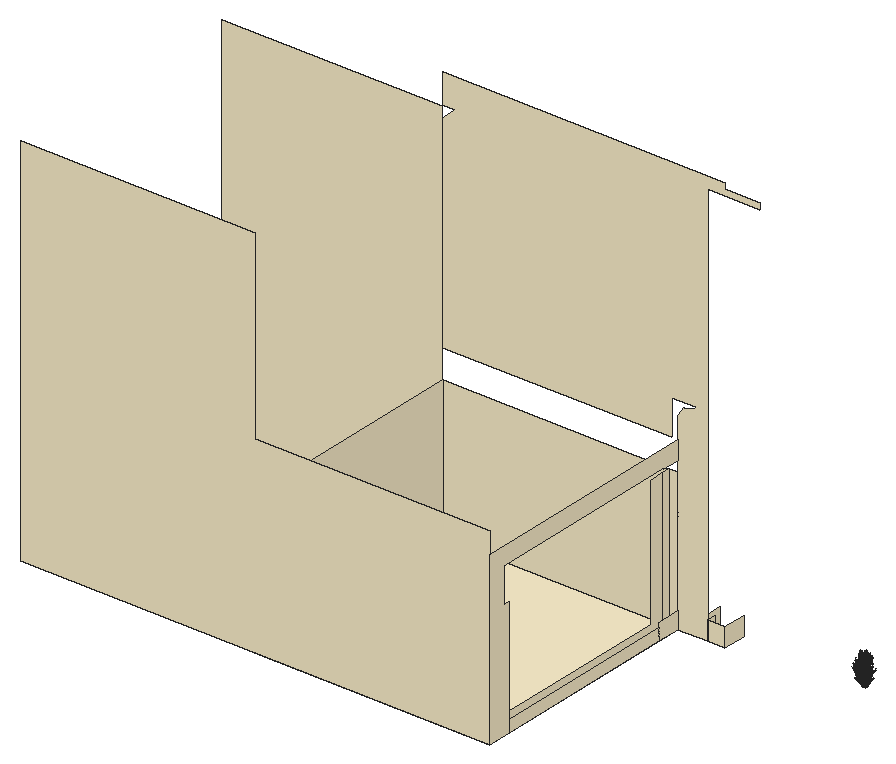
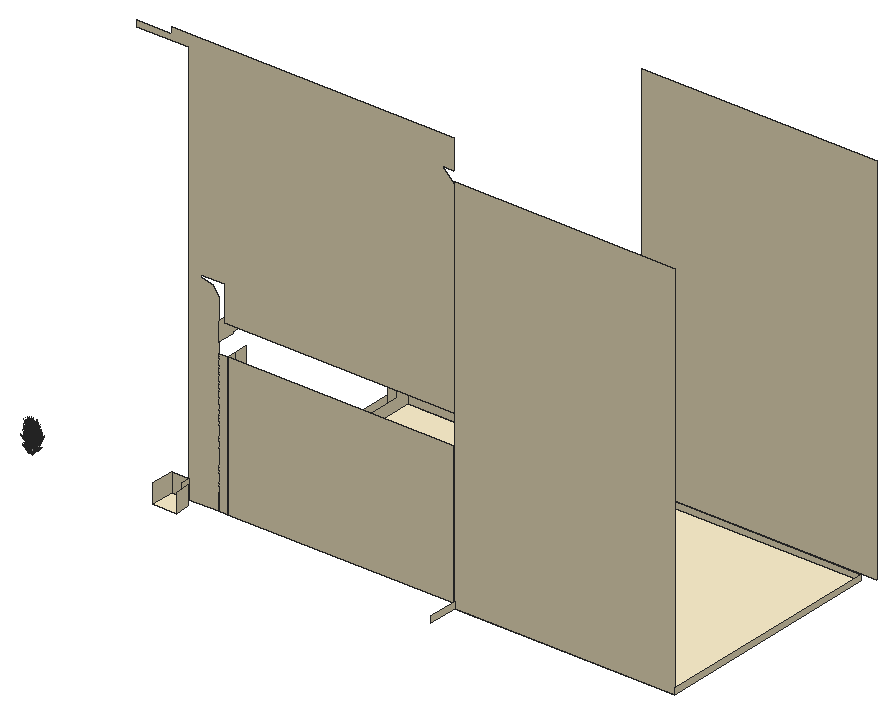
# SketchUp Ruby script. Lengths in inches.
U = 1.inch
M = Sketchup.active_model
def pt(a) = Geom::Point3d.new(a.map { |v| v * U })
def face(e, loops, mat)
  f = e.add_face(loops[0].map { |a| pt(a) })
  loops[1..].each { |l| e.add_face(l.map { |a| pt(a) }).erase! }
  f.material = f.back_material = mat if mat
  f
end
# faces: each face lists its corners as indices into pts; further lists are holes
def faces(e, pts, list, mat = nil) = list.each { |f| face(e, (f[0].is_a?(Array) ? f : [f]).map { |l| l.map { |i| pts[i] } }, mat) }
# xy, xz, yz: faces in a plane at the given z, y or x. An outline is a flat list of corners, or four numbers for a rectangle; further outlines are holes
def ring(l) = l.size == 4 ? [[l[0], l[1]], [l[2], l[1]], [l[2], l[3]], [l[0], l[3]]] : l.each_slice(2).to_a
def flat(e, list, mat, &to3) = list.each { |f| face(e, (f[0].is_a?(Array) ? f : [f]).map { |l| ring(l).map { |u, v| to3.(u, v) } }, mat) }
def xy(e, z, list, mat = nil) = flat(e, list, mat) { |x, y| [x, y, z] }
def xz(e, y, list, mat = nil) = flat(e, list, mat) { |x, z| [x, y, z] }
def yz(e, x, list, mat = nil) = flat(e, list, mat) { |y, z| [x, y, z] }
def lines(e, pts, list) = list.each { |a, b| e.add_line(pt(pts[a]), pt(pts[b])) }
# prism: a flat outline (further loops are holes) pulled along v
def prism(e, loops, v, mat = nil)
  f = face(e, loops, mat); d = Geom::Vector3d.new(v.map { |x| x * U })
  f.pushpull(f.normal.samedirection?(d) ? d.length : -d.length)
end
def box(e, o, s, mat = nil) = prism(e, [[o, [o[0] + s[0], o[1], o[2]], [o[0] + s[0], o[1] + s[1], o[2]], [o[0], o[1] + s[1], o[2]]]], [0, 0, s[2]], mat)
def at(x, y, z, deg = 0) = Geom::Transformation.translation(pt([x, y, z])) * Geom::Transformation.rotation(ORIGIN, Z_AXIS, deg.degrees)
def axes(o, x, y, z) = Geom::Transformation.new([*x, 0, *y, 0, *z, 0, *pt(o).to_a, 1])
def part(name) = M.definitions.add(name)
# library, detail: a bought-in or finely detailed component or shape, given as its bounding box
def library(name, o, s) = part(name).tap { |d| box(d.entities, o, s) }
def detail(e, o, s) = box(e.add_group.entities, o, s)
def put(e, d, t, mat = nil) = e.add_instance(d, t).tap { |i| i.material = mat if mat }
def group(e, t, mat = nil) = e.add_group.tap { |g| g.transformation = t; g.material = mat if mat }.entities
root = M.entities
M.materials.add("D01_Frost_White").color = [255, 242, 206]
M.materials.add("LightPink_Translucent").color = [144, 107, 117]
M.materials["LightPink_Translucent"].alpha = 0.75
c1 = part("blade")
p = [[2.15,0.21,22],[0,0.17,0],[0.09,0.45,0],[2.18,0.31,22],[2.29,0.31,22],[0.38,0.45,0],
  [2.48,0.24,33],[2.49,0.24,33],[2.48,0.22,33]]
faces(c1.entities,p,[[0,1,2,3],[4,5,2,3],[6,3,4,7],[8,0,3,6]])
c2 = part("seeds")
p = [[0.3,-0.1,1.38],[-0.01,-0.03,1.59],[-0.01,-0.03,0.03],[0.14,-0.07,-0.07],[0.29,-0.03,3],[0.15,0.01,3.11]]
faces(c2.entities,p,[[0,1,2,3],[1,0,4,5]],"LightPink_Translucent")
c3 = part("blade with seeds")
put(c3.entities,c1,at(0,0,0))
put(c3.entities,c2,axes([2.4,0.25,30.99],[1.5799,-0.05474,1.17369],[-0.12525,1.92788,0.29478],[-0.07173,-0.02425,1.56792]))
xy(root,0,[[252,18,252,27,483,27,483,258,492,258,492,18],[21,27,21,264,246,264,246,258,243,258,243,27],[252,27,483,258],[522,258,522,267,516,267,516,282,540.12,282,540.12,258]],"D01_Frost_White")
xz(root,18,[[12,0,492,0,492,196,252,196,252,384,12,384]],"D01_Frost_White")
xz(root,27,[[21,0,243,6],[252,0,261,144],[261,0,483,144]],"D01_Frost_White")
xz(root,258,[[243,0,246,6],[252,0,483,144],[492,0,522,0,522,414,576,414,576,420,540,420,540,426,252,426,252,396.02,258.49,396,264,396,252,384,252,174,486,174,486,210,510,210,510,208,498,205,492,196],[483,0,492,144],[522,0,540.12,19.19]],"D01_Frost_White")
xz(root,264,[[21,0,246,390]],"D01_Frost_White")
xz(root,267,[[516,0,522,9]],"D01_Frost_White")
yz(root,21,[[27,0,264,6]],"D01_Frost_White")
yz(root,243,[[27,0,258,6]],"D01_Frost_White")
yz(root,246,[[258,0,264,6],[264,0,294,6]],"D01_Frost_White")
yz(root,252,[[27,0,258,144]],"D01_Frost_White")
yz(root,483,[[27,0,27,144,42,144,42,12,234,12,234,144,249,144,249,0],[249,0,258,144]],"D01_Frost_White")
yz(root,492,[[18,0,234,0,234,12,42,12,42,120,36,120,36,156,240,156,240,154.7,258,154.7,258,174,18,174],[234,0,258,17.1875]],"D01_Frost_White")
yz(root,516,[[267,0,282,19.19]],"D01_Frost_White")
yz(root,522,[[258,0,267,19.19]],"D01_Frost_White")
yz(root,540.12,[[258,0,282,19.19]],"D01_Frost_White")
p = [[492,42,12],[492,42,0]]
lines(root,p,[[0,1]])
put(root,c3,axes([664.51,277.94,1.9375],[0.19062,-0.00741,0.85688],[-0.12645,0.32094,0.06928],[-0.27165,-0.01985,0.36631]))
put(root,c3,axes([664.59,278.51,1.9375],[0.15946,-0.06916,0.85688],[0.13424,0.31957,0.06928],[-0.25033,0.07223,0.36631]))
put(root,c3,axes([664.1,279.05,1.3],[0.15971,0.02684,0.71501],[0.10294,0.27415,-0.15377],[-0.21694,0.05132,0.3057]))
put(root,c3,axes([665.51,278.17,1.67],[0.13063,-0.0473,0.88532],[0.04505,0.33024,0.06928],[-0.28294,0.04382,0.31642]))
put(root,c3,axes([664.1,278.39,2.36],[-0.07505,0.04245,0.87472],[0.00638,0.31015,-0.13834],[-0.17202,0.04033,0.07015]))
put(root,c3,axes([665.08,277.64,2.49],[-0.45939,-0.00787,-0.35523],[0.03085,-0.3315,0.04287],[-0.19462,-0.03498,0.5025]))
put(root,c3,axes([664.71,277.72,1.3],[0.08973,0.09103,0.71501],[-0.20675,0.24743,-0.15377],[-0.2123,-0.05914,0.3057]))
put(root,c3,axes([664.35,278.22,2.26],[-0.38192,-0.09121,-0.17707],[0.11139,-0.2661,0.2286],[-0.15377,0.0244,0.4374]))
put(root,c3,axes([664.875,277.43,1.9375],[0.1707,0.05633,0.85688],[-0.35326,0.23632,0.06928],[-0.22018,-0.10661,0.36631]))
put(root,c3,axes([663.27,278.71,2.35],[0.05865,0.00877,0.88692],[0.18143,0.28888,-0.08381],[-0.12006,0.07582,0.15695]))
put(root,c3,axes([664.61,278.35,2.34],[-0.1245,0.29741,-0.25549],[-0.42685,-0.10194,-0.1979],[-0.17186,0.02727,0.48886]))
put(root,c3,axes([664.93,277.71,2.34],[-0.3337,0.21658,-0.25549],[-0.29224,-0.22879,-0.1979],[-0.16955,-0.03295,0.48886]))
put(root,c3,axes([664.39,278.33,0.75],[0.01165,0.05153,0.88171],[-0.23495,0.26909,-0.1347],[-0.16689,-0.01356,0.15018]))
put(root,c3,axes([664.46,277.1,2.35],[0.03407,0.03263,0.88692],[-0.16424,0.29331,-0.08381],[-0.16634,0.00212,0.15695]))
put(root,c3,axes([663.76,279.625,1.38],[0.19152,-0.14818,0.5743],[0.07557,0.23459,0.42196],[-0.13841,0.042,0.12649]))
put(root,c3,axes([664.84,276.91,2.36],[-0.09888,-0.00231,0.87472],[-0.3148,0.23079,-0.13834],[-0.16797,-0.04716,0.07015]))
put(root,c3,axes([664.43,278.18,2.37],[0.12984,-0.29812,0.24001],[0.42685,0.10194,0.1979],[-0.16786,0.01792,0.49665]))
put(root,c3,axes([664.59,278.1,2.52],[0.23123,0.29606,-0.0608],[-0.41039,0.14549,-0.33747],[-0.17294,0.03906,0.51278]))
put(root,c3,axes([665.11,277.48,2.52],[-0.02461,0.33251,-0.0608],[-0.4659,-0.00909,-0.33747],[-0.17944,-0.0231,0.51278]))
put(root,c3,axes([664.81,277.51,2.26],[-0.26148,-0.20471,-0.17707],[0.29857,-0.19378,0.2286],[-0.1517,-0.02948,0.4374]))
put(root,c3,axes([664.4,278.1,2.37],[-0.16879,-0.22293,0.03215],[0.30779,-0.10912,0.2531],[-0.13568,0.02153,0.38595]))
put(root,c3,axes([665.18,278.72,1.9375],[0.11478,-0.10046,0.85688],[0.28982,0.27117,0.06928],[-0.19878,0.12349,0.36631]))
put(root,c3,axes([664.49,278.98,2.26],[-0.40003,0.04673,-0.17707],[-0.10563,-0.26712,0.2286],[-0.11464,0.07175,0.4374]))
put(root,c3,axes([664.27,279.78,0.75],[0.06164,0.03267,0.88171],[0.10452,0.30266,-0.1347],[-0.13662,0.06454,0.15018]))
put(root,c3,axes([664.18,278,1.38],[0.2934,-0.0234,0.5743],[-0.18611,0.20614,0.42196],[-0.14499,-0.03092,0.12649]))
put(root,c3,axes([664.54,278.93,2.37],[-0.11397,-0.30091,0.24001],[0.44709,-0.05222,0.1979],[-0.13177,0.07077,0.49665]))
put(root,c3,axes([664.77,277.43,2.55],[0.37952,-0.24129,0.26881],[0.32731,0.25625,0.22165],[-0.17806,-0.04451,0.55625]))
put(root,c3,axes([664.45,278.87,2.37],[-0.31549,-0.13751,0.03215],[0.18368,-0.19581,0.2531],[-0.10115,0.06331,0.38595]))
put(root,c3,axes([664.75,278.1875,2.53],[0.38192,0.09121,0.17707],[-0.11139,0.2661,-0.2286],[-0.15377,0.0244,0.4374]))
put(root,c3,axes([664.81,279.01,2.34],[0.11806,0.29854,-0.25549],[-0.44709,0.05222,-0.1979],[-0.12812,0.08019,0.48886]))
put(root,c3,axes([664.94,277.43,2.37],[0.02314,-0.24862,0.03215],[0.34943,0.00682,0.2531],[-0.13385,-0.02602,0.38595]))
put(root,c3,axes([665.93,278.8,1.03],[-0.47805,-0.0536,-0.31177],[0.10088,-0.33065,-0.08182],[-0.14266,-0.04007,0.68817]))
put(root,c3,axes([666.02,277,2.72],[-0.30671,0.31344,-0.0681],[-0.44417,-0.18058,-0.37797],[-0.1544,-0.08856,0.57432]))
put(root,c3,axes([665.18,277.61,2.53],[0.26148,0.20471,0.17707],[-0.29857,0.19378,-0.2286],[-0.1517,-0.02948,0.4374]))
put(root,c3,axes([665.88,277.25,2.49],[-0.39186,-0.15803,-0.35523],[0.27849,-0.27693,0.04287],[-0.14198,-0.09436,0.5025]))
put(root,c3,axes([665.7,277.26,2.34],[-0.45348,0.07772,-0.25549],[-0.07933,-0.29434,-0.1979],[-0.1218,-0.08435,0.48886]))
put(root,c3,axes([665.3,279.43,1.01],[-0.4301,-0.16348,-0.24825],[0.25708,-0.29314,0],[-0.09796,-0.03723,0.78752]))
put(root,c3,axes([665.11,276.99,0.75],[-0.04451,0.04307,0.88171],[-0.44986,0.09286,-0.1347],[-0.10868,-0.08448,0.15018]))
put(root,c3,axes([664.6,278.8,2.52],[0.4251,0.18028,-0.0608],[-0.24491,0.26108,-0.33747],[-0.1201,0.09075,0.51278]))
put(root,c3,axes([665.5625,279.625,1.1875],[-0.28732,0.32763,0],[-0.4807,-0.18271,-0.25804],[-0.10948,-0.04161,0.81856]))
put(root,c3,axes([663.9,279.58,2.82],[0.40553,0.08728,-0.03244],[-0.12475,0.26862,-0.14708],[-0.06633,0.04078,0.48512]))
put(root,c3,axes([664.8125,278.83,2.53],[0.40003,-0.04673,0.17707],[0.10563,0.26712,-0.2286],[-0.11464,0.07175,0.4374]))
put(root,c3,axes([664.83,277.16,1.0625],[-0.13257,0.26698,-0.01946],[-0.40802,-0.08212,-0.08825],[-0.06195,-0.04367,0.29107]))
put(root,c3,axes([665.9,276.25,2.35],[-0.00857,0.03919,0.88692],[-0.42284,0.14223,-0.08381],[-0.12443,-0.0727,0.15695]))
put(root,c3,axes([665.44,276.82,1.3],[-0.02783,0.10696,0.71501],[-0.40683,0.08954,-0.15377],[-0.0951,-0.13825,0.3057]))
put(root,c3,axes([665.58,277.1,1.9375],[0.10505,0.10498,0.85688],[-0.48542,0.08838,0.06928],[-0.10971,-0.1648,0.36631]))
put(root,c3,axes([666.47,278.85,1.33],[-0.46399,0.21707,-0.14548],[-0.30855,-0.30672,-0.25001],[-0.11448,-0.03115,0.79854]))
put(root,c3,axes([665.75,277.04,2.26],[-0.07098,-0.26335,-0.17707],[0.40574,-0.06954,0.2286],[-0.10898,-0.07547,0.4374]))
put(root,c3,axes([664.61,278.375,1.1875],[-0.57465,0,0],[0,-0.36542,-0.25804],[0,-0.08323,0.81856]))
put(root,c3,axes([665.42,279.3,1.01],[-0.10795,-0.28489,-0.15489],[0.42874,-0.0809,0.15489],[-0.08643,-0.03285,0.69487]))
put(root,c3,axes([665.07,279.51,2.37],[-0.37765,-0.01523,0.03215],[0.01035,-0.23004,0.2531],[-0.03952,0.08812,0.38595]))
put(root,c3,axes([666.78,279.09,1.03],[-0.30954,0.24575,-0.31177],[-0.38452,-0.22284,-0.08182],[-0.12404,0.0613,0.68817]))
put(root,c3,axes([665.99,277.26,2.53],[0.07098,0.26335,0.17707],[-0.40574,0.06954,-0.2286],[-0.10898,-0.07547,0.4374]))
put(root,c3,axes([665.06,278.28,1.17],[-0.42746,0.27488,0.15378],[-0.42772,-0.27199,-0.18246],[-0.01493,-0.07806,0.82443]))
put(root,c3,axes([666.82,279.04,1.66],[0.39713,0.13184,0.7563],[-0.38905,0.28403,0.29908],[-0.17427,-0.16834,0.63403]))
put(root,c3,axes([665.3,276.65,1.38],[0.23972,0.1138,0.5743],[-0.34912,0.06841,0.42196],[-0.0747,-0.08746,0.12649]))
put(root,c3,axes([666.99,278.95,1.23],[-0.44875,-0.26316,-0.12596],[0.3776,-0.2955,0.27565],[-0.12084,0.03078,0.84108]))
put(root,c3,axes([666.18,278.7,1.11],[-0.27607,-0.27443,-0.2237],[0.41817,-0.19325,0.10766],[-0.08934,-0.03396,0.71822]))
put(root,c3,axes([665.8,276.95,2.55],[0.51193,-0.08404,0.26881],[0.08885,0.32966,0.22165],[-0.1204,-0.09716,0.55625]))
put(root,c3,axes([666.77,278.89,1.11],[-0.49904,0.02018,-0.2237],[-0.04513,-0.33504,0.10766],[-0.08934,0.03396,0.71822]))
put(root,c3,axes([665.92,277.02,2.37],[0.20887,-0.2077,0.03215],[0.29744,0.12092,0.2531],[-0.09616,-0.06659,0.38595]))
put(root,c3,axes([665.8125,279.45,1.24],[0.4301,0.16348,0.24825],[-0.25708,0.29314,0],[-0.09796,-0.03723,0.78752]))
put(root,c3,axes([666.22,278.85,1.22],[0.1218,-0.38743,-0.11714],[0.57753,0.06753,0.25635],[-0.10091,-0.0535,0.7822]))
put(root,c3,axes([666.43,278.94,1.31],[-0.08866,0.29179,0.0724],[-0.43315,-0.05065,-0.20674],[-0.07883,-0.02996,0.63372]))
put(root,c3,axes([666.38,276.4,2.36],[-0.07029,-0.04584,0.87472],[-0.46908,0.02906,-0.13834],[-0.07486,-0.10965,0.07015]))
put(root,c3,axes([667.29,279.76,1.01],[-0.4301,0.16348,-0.24825],[-0.25708,-0.29314,0],[-0.09796,0.03723,0.78752]))
put(root,c3,axes([664.74,278.13,1.01],[0,-0.32696,-0.24825],[0.51416,0,0],[0,-0.07447,0.78752]))
put(root,c3,axes([664.96,278.43,1.24],[0,0.32696,0.24825],[-0.51416,0,0],[0,-0.07447,0.78752]))
put(root,c3,axes([667.32,279.67,1.1],[-0.28374,-0.32877,-0.02571],[0.4807,-0.18271,0.25804],[-0.11845,0.0313,0.81815]))
put(root,c3,axes([667.1875,279.63,1.01],[-0.42874,-0.0809,-0.15489],[0.10795,-0.28489,0.15489],[-0.08643,0.03285,0.69487]))
put(root,c3,axes([665.35,279.36,2.53],[0.31095,-0.17214,0.17707],[0.29435,0.19656,-0.2286],[-0.04479,0.09987,0.4374]))
put(root,c3,axes([666.09,278.51,1.33],[-0.51755,-0.15601,-0.14548],[0.2492,-0.32927,-0.25001],[-0.01626,-0.08084,0.79854]))
put(root,c3,axes([667.44,278.41,1.42],[-0.01255,-0.30784,0.70636],[0.56816,0.0798,0.29908],[-0.13438,0.16845,0.66675]))
put(root,c3,axes([667.12,278.8,1.33],[0.05355,0.37308,-0.14548],[-0.55775,0.02256,-0.25001],[-0.09822,0.04969,0.79854]))
put(root,c3,axes([665.86,278.17,1.05],[-0.18873,-0.33528,-0.34918],[0.54365,-0.12075,-0.09164],[-0.02086,-0.11353,0.77075]))
put(root,c3,axes([667.09,277.11,2.52],[-0.44971,0.15222,-0.0608],[-0.221,-0.27017,-0.33747],[-0.05933,-0.11385,0.51278]))
put(root,c3,axes([666.71,277.12,2.34],[-0.45175,-0.08196,-0.25549],[0.15485,-0.28101,-0.1979],[-0.04142,-0.11314,0.48886]))
put(root,c3,axes([664.96,278.14,1.01],[0.32079,-0.20399,-0.15489],[0.32079,0.20399,0.15489],[0,-0.06571,0.69487]))
put(root,c3,axes([666.41,276.82,1.0625],[-0.31757,0.18757,-0.01946],[-0.29098,-0.20543,-0.08825],[-0.02049,-0.05821,0.29107]))
put(root,c3,axes([666.28,278.67,1.18],[0.58084,0.06889,0.22877],[-0.11821,0.38906,0.08977],[-0.08488,-0.03757,0.79428]))
put(root,c3,axes([666.13,278.6,1.36],[-0.22297,0.29461,0.2237],[-0.4633,-0.14179,-0.10766],[0,-0.06791,0.71822]))
put(root,c3,axes([666.87,277.18,2.49],[-0.21934,-0.26585,-0.35523],[0.45151,-0.14816,0.04287],[-0.05129,-0.12845,0.5025]))
put(root,c3,axes([665.97,279.29,1.24],[0.49383,-0.08678,0.08821],[0.12194,0.32295,0.17543],[-0.04404,-0.04705,0.80203]))
put(root,c3,axes([666.61,279.34,1.1],[-0.4633,-0.14679,0],[0.22297,-0.30501,0],[0,0,0.81353]))
put(root,c3,axes([666.96,277.22,2.53],[-0.13855,0.25143,0.17707],[-0.4042,-0.07334,-0.2286],[-0.03706,-0.10123,0.4374]))
put(root,c3,axes([667.68,279.71,1.1875],[0.28732,0.32763,0],[-0.4807,0.18271,-0.25804],[-0.10948,0.04161,0.81856]))
put(root,c3,axes([667.44,279.31,1.24],[0.13276,-0.32494,0.08821],[0.4858,0.09195,0.17543],[-0.08392,0.00158,0.80203]))
put(root,c3,axes([667.22,278.875,1.31],[0.33952,0.19644,0.0724],[-0.2832,0.22163,-0.20674],[-0.07883,0.02996,0.63372]))
put(root,c3,axes([667.1,278.63,1.15],[-0.42746,-0.28142,-0.03066],[0.42772,-0.28159,0],[-0.01493,-0.00983,0.87786]))
put(root,c3,axes([667.21,278.73,1.36],[0.49904,-0.02018,0.2237],[0.04513,0.33504,-0.10766],[-0.08934,0.03396,0.71822]))
put(root,c3,axes([667.33,279.5,1.17],[0.57533,0.10627,0.15378],[-0.14394,0.37986,-0.18246],[-0.09522,0.04754,0.82443]))
put(root,c3,axes([666.49,276.59,0.75],[-0.07708,0.01178,0.88171],[-0.42627,-0.1326,-0.1347],[0.00715,-0.1106,0.15018]))
put(root,c3,axes([667.58,279.48,1.24],[0.4301,-0.16348,0.24825],[0.25708,0.29314,0],[-0.09796,0.03723,0.78752]))
put(root,c3,axes([666.91,276.95,2.26],[0.13855,-0.25143,-0.17707],[0.4042,0.07334,0.2286],[-0.03706,-0.10123,0.4374]))
put(root,c3,axes([666.23,278.31,1.18],[0.1998,0.3656,0.22877],[-0.5709,0.12713,0.08977],[0.00698,-0.06718,0.79428]))
put(root,c3,axes([666.14,278.26,1.11],[0.22297,-0.29461,-0.2237],[0.4633,0.14179,0.10766],[0,-0.06791,0.71822]))
put(root,c3,axes([666.71,279.21,1.1],[-0.14994,-0.28188,0],[0.42817,-0.09871,0],[0,0,0.77185]))
put(root,c3,axes([667.32,278.66,1.11],[-0.22297,0.29461,-0.2237],[-0.4633,-0.14179,0.10766],[0,0.06791,0.71822]))
put(root,c3,axes([667.08,276.99,2.37],[0.33863,-0.11112,0.03215],[0.16575,0.20263,0.2531],[-0.0327,-0.08932,0.38595]))
put(root,c3,axes([668.2,278.48,1.24],[-0.36107,-0.23816,0.08821],[0.36387,-0.231,0.17543],[-0.03988,0.04864,0.80203]))
put(root,c3,axes([666.95,278.34,1.1],[0,-0.37831,0],[0.57465,0,0],[0,0,0.89728]))
put(root,c3,axes([666.96,277.01,2.37],[0.45283,0.08548,0.24001],[-0.15485,0.28101,0.1979],[-0.02721,-0.11051,0.49665]))
put(root,c3,axes([666.42,278.41,1.22],[0.5178,0.15847,0.12032],[-0.2492,0.32927,0.25001],[0,-0.0759,0.80271]))
put(root,c3,axes([667.24,278.49,1.15],[0,0.37813,-0.02818],[-0.57465,0,0],[0,0.01188,0.89684]))
put(root,c3,axes([666.25,278.1875,1.36],[-0.49904,0.02018,0.2237],[-0.04513,-0.33504,-0.10766],[0.08934,-0.03396,0.71822]))
put(root,c3,axes([666.02,277.61,1.24],[-0.13276,0.32494,0.08821],[-0.4858,-0.09195,0.17543],[0.08392,-0.00158,0.80203]))
put(root,c3,axes([666.97,279.22,1.15],[0.1998,0.37562,-0.03006],[-0.5709,0.13162,0],[0.00698,0.01312,0.86086]))
put(root,c3,axes([665.78,277.21,1.1875],[-0.28732,-0.32763,0],[0.4807,-0.18271,-0.25804],[0.10948,-0.04161,0.81856]))
put(root,c3,axes([668.62,278.73,1.1],[-0.57436,-0.00261,-0.02488],[0,-0.36542,0.24971],[-0.01805,0.08319,0.79176]))
put(root,c3,axes([667.49,277.63,1.24],[-0.49383,0.08678,0.08821],[-0.12194,-0.32295,0.17543],[0.04404,0.04705,0.80203]))
put(root,c3,axes([666.98,276.42,1.38],[0.05895,0.19066,0.5743],[-0.32704,-0.1056,0.42196],[0.03519,-0.09762,0.12649]))
put(root,c3,axes([666.68,278.1,1.18],[-0.38104,0.29672,0.22877],[-0.45269,-0.26192,0.08977],[0.09186,-0.02961,0.79428]))
put(root,c3,axes([667.33,278.57,1.11],[0.32079,0.21119,0],[-0.32079,0.21119,0],[0,0,0.84633]))
put(root,c3,axes([667.33,278.32,1.36],[0.22297,-0.29461,0.2237],[0.4633,0.14179,-0.10766],[0,0.06791,0.71822]))
put(root,c3,axes([667.13,279.34,1.1],[0.4633,0.14679,0],[-0.22297,0.30501,0],[0,0,0.87477]))
put(root,c3,axes([667.18,278.25,1.19],[-0.58084,-0.06889,0.24599],[0.11821,-0.38906,0.09653],[0.08488,0.03757,0.85407]))
put(root,c3,axes([668.39,276.73,2.35],[-0.04667,0.02497,0.88692],[-0.45726,-0.08426,-0.08381],[-0.01655,-0.10898,0.15695]))
put(root,c3,axes([668.03,277.45,2.52],[-0.50507,-0.0162,-0.0608],[0.01381,-0.30672,-0.33747],[0.03508,-0.11813,0.51278]))
put(root,c3,axes([668.5,278.78,1.01],[-0.32079,0.20399,-0.15489],[-0.32079,-0.20399,0.15489],[0,0.06571,0.69487]))
put(root,c3,axes([667.58,278.74,1.05],[0.16851,0.29936,-0.34606],[-0.4854,0.10781,-0.09083],[0.01863,0.10137,0.76386]))
put(root,c3,axes([667.34,278.42,1.1],[0.51416,0,0],[0,0.33849,0],[0,0,0.89203]))
put(root,c3,axes([667.83,277.5,2.53],[-0.31095,0.17214,0.17707],[-0.29435,-0.19656,-0.2286],[0.04479,-0.09987,0.4374]))
put(root,c3,axes([666.85,278.05,1.36],[-0.27607,-0.27443,0.2237],[0.41817,-0.19325,-0.10766],[0.08934,0.03396,0.71822]))
put(root,c3,axes([666.35,278.12,1.33],[-0.05355,-0.37308,-0.14548],[0.55775,-0.02256,-0.25001],[0.09822,-0.04969,0.79854]))
put(root,c3,axes([667.52,278.39,1.31],[0.42817,-0.09535,0.0724],[0.14994,0.27228,-0.20674],[0,0.05992,0.63372]))
put(root,c3,axes([667.68,277.34,2.34],[-0.32898,-0.21969,-0.25549],[0.34753,-0.1924,-0.1979],[0.05006,-0.11162,0.48886]))
put(root,c3,axes([667.375,278.41,1.33],[0.51755,0.15601,-0.14548],[-0.2492,0.32927,-0.25001],[0.01626,0.08084,0.79854]))
put(root,c3,axes([666.27,277.29,1.01],[0.42874,0.0809,-0.15489],[-0.10795,0.28489,0.15489],[0.08643,-0.03285,0.69487]))
put(root,c3,axes([667.47,276.95,1.3],[-0.13063,0.06618,0.71501],[-0.39122,-0.11583,-0.15377],[0.07252,-0.14406,0.3057]))
put(root,c3,axes([668.5,278.49,1.24],[0,-0.32696,0.24825],[0.51416,0,0],[0,0.07447,0.78752]))
put(root,c3,axes([668.72,278.79,1.01],[0,0.32696,-0.24825],[-0.51416,0,0],[0,0.07447,0.78752]))
put(root,c3,axes([666.17,277.16,1.01],[0.4301,-0.16348,-0.24825],[0.25708,0.29314,0],[0.09796,-0.03723,0.78752]))
put(root,c3,axes([667.03,277.97,1.31],[0.08866,-0.29179,0.0724],[0.43315,0.05065,-0.20674],[0.07883,0.02996,0.63372]))
put(root,c3,axes([667.65,277.46,1.24],[-0.4301,-0.16348,0.24825],[0.25708,-0.29314,0],[0.09796,0.03723,0.78752]))
put(root,c3,axes([667.78,277.4375,2.49],[0.01196,-0.30243,-0.35523],[0.50354,0.02031,0.04287],[0.05314,-0.12813,0.5025]))
put(root,c3,axes([667.28,279.17,1.09],[0.48247,-0.11094,-0.09599],[0.16954,0.31956,0.00004],[0.05326,-0.01226,0.86949]))
put(root,c3,axes([667.19,279.6,2.53],[-0.07098,-0.26335,0.17707],[0.40574,-0.06954,-0.2286],[0.10898,0.07547,0.4374]))
put(root,c3,axes([667.28,278.22,1.11],[0.27607,0.27443,-0.2237],[-0.41817,0.19325,0.10766],[0.08934,0.03396,0.71822]))
put(root,c3,axes([667.47,278.08,2.24],[-0.39711,-0.16988,0.69141],[0.41931,-0.2645,0.29833],[0.12812,0.1594,0.66832]))
put(root,c3,axes([667.99,277.25,2.26],[0.31095,-0.17214,-0.17707],[0.29435,0.19656,0.2286],[0.04479,-0.09987,0.4374]))
put(root,c3,axes([666.8,279.97,2.35],[0.00136,-0.03958,0.88692],[0.39383,-0.17464,-0.08381],[0.1368,0.06234,0.15695]))
put(root,c3,axes([668.11,277.34,2.37],[0.37765,0.01523,0.03215],[-0.01035,0.23004,0.2531],[0.03952,-0.08812,0.38595]))
put(root,c3,axes([668.07,279.47,1.38],[-0.25875,-0.09401,0.5743],[0.33411,-0.09552,0.42196],[0.09012,0.08091,0.12649]))
put(root,c3,axes([668.49,276.96,2.36],[-0.00444,-0.06507,0.87472],[-0.37468,-0.18807,-0.13834],[0.05793,-0.114,0.07015]))
put(root,c3,axes([666.68,277.83,1.03],[0.30954,-0.24575,-0.31177],[0.38452,0.22284,-0.08182],[0.12404,-0.0613,0.68817]))
put(root,c3,axes([667.99,277.32,2.37],[0.32725,0.22308,0.24001],[-0.34753,0.1924,0.1979],[0.06036,-0.10466,0.49665]))
put(root,c3,axes([668.04,277.61,1.01],[0.10795,0.28489,-0.15489],[-0.42874,0.0809,0.15489],[0.08643,0.03285,0.69487]))
put(root,c3,axes([668.85,278.54,1.1875],[0.57465,0,0],[0,0.36542,-0.25804],[0,0.08323,0.81856]))
put(root,c3,axes([666.99,278.07,1.33],[0.46399,-0.21707,-0.14548],[0.30855,0.30672,-0.25001],[0.11448,0.03115,0.79854]))
put(root,c3,axes([668.37,278.03,2.53],[-0.40003,0.04673,0.17707],[-0.10563,-0.26712,-0.2286],[0.11464,-0.07175,0.4374]))
put(root,c3,axes([667.22,277.28,1.9375],[-0.08557,0.11238,0.85688],[-0.35897,-0.23257,0.06928],[0.16194,-0.14495,0.36631]))
put(root,c3,axes([667.16,279.74,2.52],[0.27385,-0.27986,-0.0608],[0.39658,0.16123,-0.33747],[0.13785,0.07907,0.51278]))
put(root,c3,axes([665.82,277.875,0.8],[-0.45234,0.1309,0.64464],[-0.14398,-0.37559,0.25048],[0.27777,0.00625,0.73321]))
put(root,c3,axes([668.58,278.05,2.52],[-0.4251,-0.18028,-0.0608],[0.24491,-0.26108,-0.33747],[0.1201,-0.09075,0.51278]))
put(root,c3,axes([667.9,277.29,1.1875],[0.28732,-0.32763,0],[0.4807,0.18271,-0.25804],[0.10948,0.04161,0.81856]))
put(root,c3,axes([668.38,277.15,0.75],[-0.06878,-0.02576,0.88171],[-0.17668,-0.28776,-0.1347],[0.11919,-0.07809,0.15018]))
put(root,c3,axes([668,279.24,2.53],[-0.26148,-0.20471,0.17707],[0.29857,-0.19378,-0.2286],[0.1517,0.02948,0.4374]))
put(root,c3,axes([668.16,277.49,1.01],[0.4301,0.16348,-0.24825],[-0.25708,0.29314,0],[0.09796,0.03723,0.78752]))
put(root,c3,axes([668.24,279.43,2.37],[-0.02314,0.24862,0.03215],[-0.34943,-0.00682,0.2531],[0.13385,0.02602,0.38595]))
put(root,c3,axes([668.14,279.82,0.75],[0.03348,-0.0472,0.88171],[0.42153,-0.13902,-0.1347],[0.12779,0.07195,0.15018]))
put(root,c3,axes([668.27,279.35,2.37],[-0.33886,0.21544,0.24001],[-0.29224,-0.22879,0.1979],[0.15898,0.03974,0.49665]))
put(root,c3,axes([668.36,277.84,2.34],[-0.11806,-0.29854,-0.25549],[0.44709,-0.05222,-0.1979],[0.12812,-0.08019,0.48886]))
put(root,c3,axes([669.15,279.38,1.96],[-0.08796,-0.27485,-0.01746],[0.41573,-0.06319,-0.07916],[0.08682,0.01742,0.26109]))
put(root,c3,axes([668.43,278.67,2.53],[-0.38192,-0.09121,0.17707],[0.11139,-0.2661,-0.2286],[0.15377,-0.0244,0.4374]))
put(root,c3,axes([667.53,278.12,1.03],[0.47805,0.0536,-0.31177],[-0.10088,0.33065,-0.08182],[0.14266,0.04007,0.68817]))
put(root,c3,axes([669.57,278.3125,1.13],[-0.28491,-0.20907,-0.03244],[0.31204,-0.19157,-0.14708],[0.08842,-0.01349,0.48512]))
put(root,c3,axes([668.91,277.25,1.38],[-0.15307,0.16644,0.5743],[-0.13157,-0.22361,0.42196],[0.12643,-0.05603,0.12649]))
put(root,c3,axes([668.73,277.99,2.37],[0.31549,0.13751,0.03215],[-0.18368,0.19581,0.2531],[0.10115,-0.06331,0.38595]))
put(root,c3,axes([668.64,277.93,2.37],[0.11397,0.30091,0.24001],[-0.44709,0.05222,0.1979],[0.13177,-0.07077,0.49665]))
put(root,c3,axes([667.43,278.83,1.9375],[-0.1707,-0.05633,0.85688],[0.35326,-0.23632,0.06928],[0.22018,0.10661,0.36631]))
put(root,c3,axes([669.62,277.98,2.35],[-0.06002,-0.00248,0.88692],[-0.24926,-0.26607,-0.08381],[0.1001,-0.08748,0.15695]))
